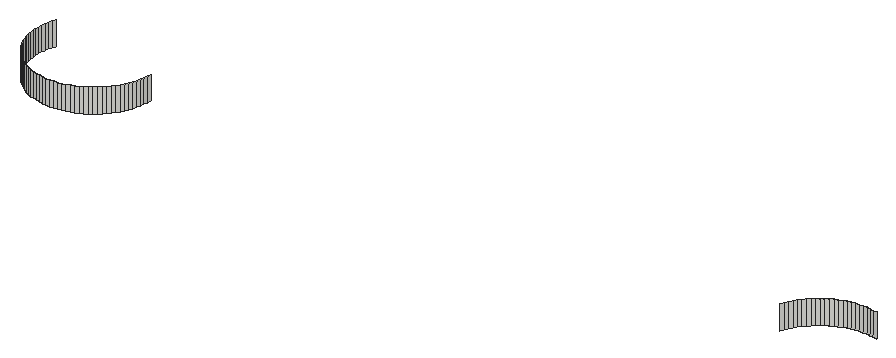
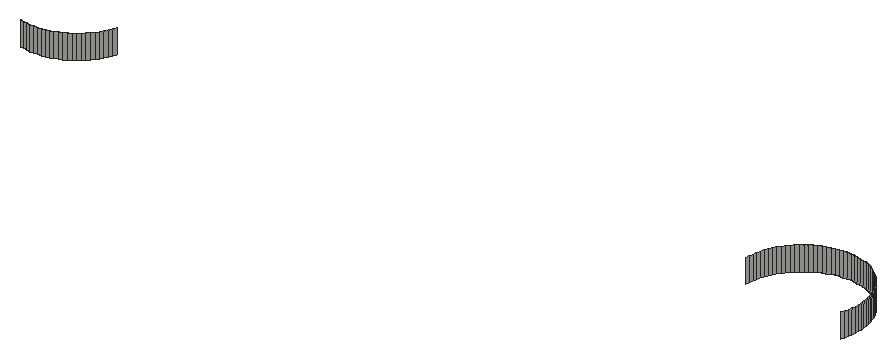
# SketchUp Ruby script. Lengths in inches.
U = 1.inch
M = Sketchup.active_model
def pt(a) = Geom::Point3d.new(a.map { |v| v * U })
def face(e, loops, mat)
  f = e.add_face(loops[0].map { |a| pt(a) })
  loops[1..].each { |l| e.add_face(l.map { |a| pt(a) }).erase! }
  f.material = f.back_material = mat if mat
  f
end
# faces: each face lists its corners as indices into pts; further lists are holes
def faces(e, pts, list, mat = nil) = list.each { |f| face(e, (f[0].is_a?(Array) ? f : [f]).map { |l| l.map { |i| pts[i] } }, mat) }
# xy, xz, yz: faces in a plane at the given z, y or x. An outline is a flat list of corners, or four numbers for a rectangle; further outlines are holes
def ring(l) = l.size == 4 ? [[l[0], l[1]], [l[2], l[1]], [l[2], l[3]], [l[0], l[3]]] : l.each_slice(2).to_a
def flat(e, list, mat, &to3) = list.each { |f| face(e, (f[0].is_a?(Array) ? f : [f]).map { |l| ring(l).map { |u, v| to3.(u, v) } }, mat) }
def xy(e, z, list, mat = nil) = flat(e, list, mat) { |x, y| [x, y, z] }
def xz(e, y, list, mat = nil) = flat(e, list, mat) { |x, z| [x, y, z] }
def yz(e, x, list, mat = nil) = flat(e, list, mat) { |y, z| [x, y, z] }
def lines(e, pts, list) = list.each { |a, b| e.add_line(pt(pts[a]), pt(pts[b])) }
# prism: a flat outline (further loops are holes) pulled along v
def prism(e, loops, v, mat = nil)
  f = face(e, loops, mat); d = Geom::Vector3d.new(v.map { |x| x * U })
  f.pushpull(f.normal.samedirection?(d) ? d.length : -d.length)
end
def box(e, o, s, mat = nil) = prism(e, [[o, [o[0] + s[0], o[1], o[2]], [o[0] + s[0], o[1] + s[1], o[2]], [o[0], o[1] + s[1], o[2]]]], [0, 0, s[2]], mat)
def at(x, y, z, deg = 0) = Geom::Transformation.translation(pt([x, y, z])) * Geom::Transformation.rotation(ORIGIN, Z_AXIS, deg.degrees)
def axes(o, x, y, z) = Geom::Transformation.new([*x, 0, *y, 0, *z, 0, *pt(o).to_a, 1])
def part(name) = M.definitions.add(name)
# library, detail: a bought-in or finely detailed component or shape, given as its bounding box
def library(name, o, s) = part(name).tap { |d| box(d.entities, o, s) }
def detail(e, o, s) = box(e.add_group.entities, o, s)
def put(e, d, t, mat = nil) = e.add_instance(d, t).tap { |i| i.material = mat if mat }
def group(e, t, mat = nil) = e.add_group.tap { |g| g.transformation = t; g.material = mat if mat }.entities
root = M.entities
xz(root,34,[[144.99,231.53,145.37,234]])
xz(root,46,[[220.18,231.53,220.56,234]])
yz(root,139.18,[[39.8125,231.53,40.1875,234]])
p = [[144.62,34.03,231.53],[144.24,34.07,231.53],[144.24,34.07,234],[144.62,34.03,234],[144.99,34,231.53],[144.99,34,234],
  [145.75,34.03,231.53],[145.37,34,231.53],[145.37,34,234],[145.75,34.03,234],[146.12,34.07,231.53],[146.12,34.07,234],
  [143.87,34.14,231.53],[143.51,34.24,231.53],[143.51,34.24,234],[143.87,34.14,234],[146.49,34.14,231.53],[146.49,34.14,234],
  [146.86,34.24,231.53],[146.86,34.24,234],[143.15,34.35,231.53],[143.15,34.35,234],[147.21,34.35,231.53],[147.21,34.35,234],
  [142.8,34.49,231.53],[142.8,34.49,234],[147.5625,34.49,231.53],[147.5625,34.49,234],[142.46,34.65,231.53],[142.46,34.65,234],
  [147.91,34.65,231.53],[147.91,34.65,234],[142.125,34.84,231.53],[142.125,34.84,234],[148.24,34.84,231.53],[148.24,34.84,234],
  [141.81,35.04,231.53],[141.81,35.04,234],[148.55,35.04,231.53],[148.55,35.04,234],[141.5,35.26,231.53],[141.5,35.26,234],
  [148.86,35.26,231.53],[148.86,35.26,234],[141.21,35.5,231.53],[141.21,35.5,234],[149.15,35.5,231.53],[149.15,35.5,234],
  [140.9375,35.76,231.53],[140.9375,35.76,234],[149.42,35.76,231.53],[149.42,35.76,234],[140.68,36.03,231.53],[140.68,36.03,234],
  [149.68,36.03,231.53],[149.68,36.03,234],[140.44,36.32,231.53],[140.44,36.32,234],[149.92,36.32,231.53],[149.92,36.32,234],
  [140.22,36.63,231.53],[140.22,36.63,234],[150.14,36.63,231.53],[150.14,36.63,234],[140.02,36.95,231.53],[140.02,36.95,234],
  [150.35,36.95,231.53],[150.35,36.95,234],[139.84,37.28,231.53],[139.84,37.28,234],[150.53,37.28,231.53],[150.53,37.28,234],
  [139.67,37.62,231.53],[139.67,37.62,234],[150.6875,37.62,231.53],[150.6875,37.62,234],[139.54,37.97,231.53],[139.54,37.97,234],
  [150.83,37.97,231.53],[150.83,37.97,234],[139.42,38.33,231.53],[139.42,38.33,234],[150.94,38.33,231.53],[150.94,38.33,234],
  [139.33,38.69,231.53],[139.33,38.69,234],[151.04,38.69,231.53],[151.04,38.69,234],[139.26,39.0625,231.53],[139.26,39.0625,234],
  [151.11,39.0625,231.53],[151.11,39.0625,234],[139.21,39.44,231.53],[139.21,39.44,234],[151.15,39.44,231.53],[151.15,39.44,234],
  [139.18,39.8125,231.53],[139.18,39.8125,234],[151.18,39.8125,231.53],[151.18,39.8125,234],[139.18,40.1875,231.53],[139.21,40.56,231.53],
  [139.21,40.56,234],[139.18,40.1875,234],[139.26,40.9375,231.53],[139.26,40.9375,234],[139.33,41.31,231.53],[139.33,41.31,234],
  [139.42,41.67,231.53],[139.42,41.67,234],[139.54,42.03,231.53],[139.54,42.03,234],[214.73,42.03,231.53],[214.86,42.38,231.53],
  [214.86,42.38,234],[214.73,42.03,234],[215.02,42.72,231.53],[215.02,42.72,234],[215.21,43.05,231.53],[215.21,43.05,234],
  [215.41,43.37,231.53],[215.41,43.37,234],[215.63,43.68,231.53],[215.63,43.68,234],[215.87,43.97,231.53],[215.87,43.97,234],
  [216.13,44.24,231.53],[216.13,44.24,234],[216.4,44.5,231.53],[216.4,44.5,234],[216.69,44.74,231.53],[216.69,44.74,234],
  [217,44.96,231.53],[217,44.96,234],[217.32,45.16,231.53],[217.32,45.16,234],[217.65,45.35,231.53],[217.65,45.35,234],
  [217.99,45.51,231.53],[217.99,45.51,234],[218.34,45.65,231.53],[218.34,45.65,234],[218.7,45.76,231.53],[218.7,45.76,234],
  [219.0625,45.86,231.53],[219.0625,45.86,234],[219.43,45.93,231.53],[219.43,45.93,234],[219.81,45.97,231.53],[219.81,45.97,234],
  [220.94,45.97,231.53],[221.31,45.93,231.53],[221.31,45.93,234],[220.94,45.97,234],[221.68,45.86,231.53],[221.68,45.86,234],
  [220.18,46,231.53],[220.18,46,234],[220.56,46,231.53],[220.56,46,234]]
faces(root,p,[[0,1,2,3],[4,0,3,5],[6,7,8,9],[10,6,9,11],[12,13,14,15],[1,12,15,2],[16,10,11,17],[18,16,17,19],
  [13,20,21,14],[22,18,19,23],[20,24,25,21],[26,22,23,27],[24,28,29,25],[30,26,27,31],[28,32,33,29],[34,30,31,35],
  [32,36,37,33],[38,34,35,39],[36,40,41,37],[42,38,39,43],[40,44,45,41],[46,42,43,47],[44,48,49,45],[50,46,47,51],
  [48,52,53,49],[54,50,51,55],[52,56,57,53],[58,54,55,59],[56,60,61,57],[62,58,59,63],[60,64,65,61],[66,62,63,67],
  [64,68,69,65],[70,66,67,71],[68,72,73,69],[74,70,71,75],[72,76,77,73],[78,74,75,79],[76,80,81,77],[82,78,79,83],
  [80,84,85,81],[86,82,83,87],[84,88,89,85],[90,86,87,91],[88,92,93,89],[94,90,91,95],[92,96,97,93],[98,94,95,99],
  [100,101,102,103],[101,104,105,102],[104,106,107,105],[106,108,109,107],[108,110,111,109],[112,113,114,115],[113,116,117,114],[116,118,119,117],
  [118,120,121,119],[120,122,123,121],[122,124,125,123],[124,126,127,125],[126,128,129,127],[128,130,131,129],[130,132,133,131],[132,134,135,133],
  [134,136,137,135],[136,138,139,137],[138,140,141,139],[140,142,143,141],[142,144,145,143],[144,146,147,145],[146,148,149,147],[150,151,152,153],
  [151,154,155,152],[148,156,157,149],[158,150,153,159]])
